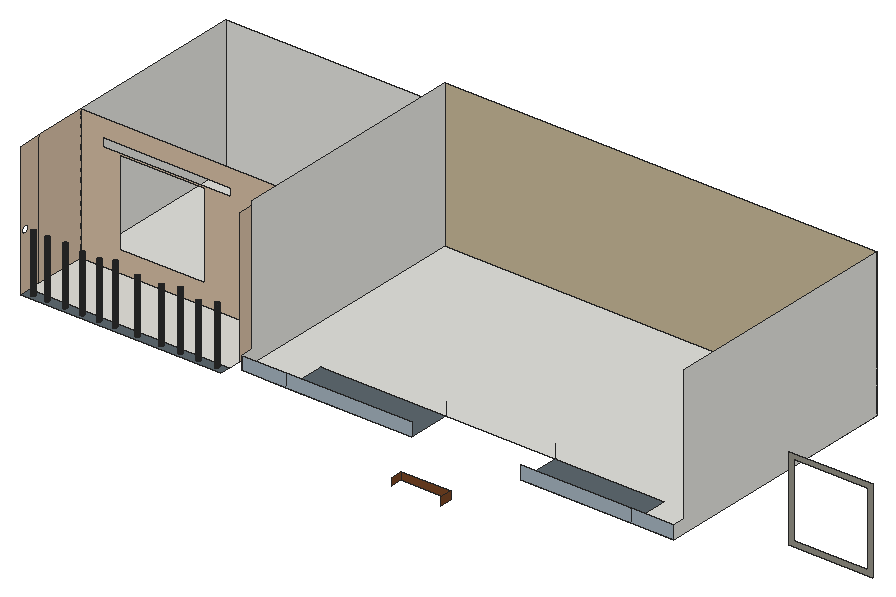
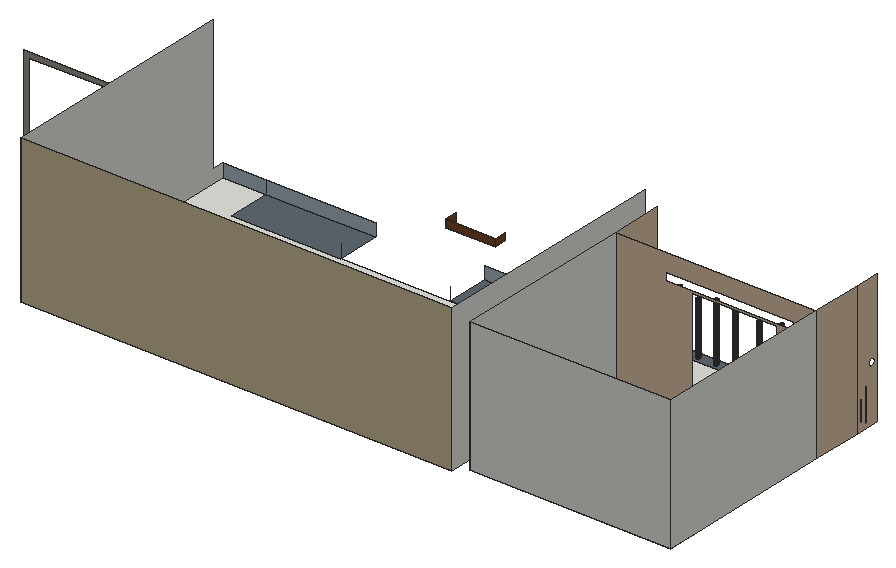
# SketchUp Ruby script. Lengths in inches.
U = 1.inch
M = Sketchup.active_model
def pt(a) = Geom::Point3d.new(a.map { |v| v * U })
def face(e, loops, mat)
  f = e.add_face(loops[0].map { |a| pt(a) })
  loops[1..].each { |l| e.add_face(l.map { |a| pt(a) }).erase! }
  f.material = f.back_material = mat if mat
  f
end
# faces: each face lists its corners as indices into pts; further lists are holes
def faces(e, pts, list, mat = nil) = list.each { |f| face(e, (f[0].is_a?(Array) ? f : [f]).map { |l| l.map { |i| pts[i] } }, mat) }
# xy, xz, yz: faces in a plane at the given z, y or x. An outline is a flat list of corners, or four numbers for a rectangle; further outlines are holes
def ring(l) = l.size == 4 ? [[l[0], l[1]], [l[2], l[1]], [l[2], l[3]], [l[0], l[3]]] : l.each_slice(2).to_a
def flat(e, list, mat, &to3) = list.each { |f| face(e, (f[0].is_a?(Array) ? f : [f]).map { |l| ring(l).map { |u, v| to3.(u, v) } }, mat) }
def xy(e, z, list, mat = nil) = flat(e, list, mat) { |x, y| [x, y, z] }
def xz(e, y, list, mat = nil) = flat(e, list, mat) { |x, z| [x, y, z] }
def yz(e, x, list, mat = nil) = flat(e, list, mat) { |y, z| [x, y, z] }
def lines(e, pts, list) = list.each { |a, b| e.add_line(pt(pts[a]), pt(pts[b])) }
# prism: a flat outline (further loops are holes) pulled along v
def prism(e, loops, v, mat = nil)
  f = face(e, loops, mat); d = Geom::Vector3d.new(v.map { |x| x * U })
  f.pushpull(f.normal.samedirection?(d) ? d.length : -d.length)
end
def box(e, o, s, mat = nil) = prism(e, [[o, [o[0] + s[0], o[1], o[2]], [o[0] + s[0], o[1] + s[1], o[2]], [o[0], o[1] + s[1], o[2]]]], [0, 0, s[2]], mat)
def at(x, y, z, deg = 0) = Geom::Transformation.translation(pt([x, y, z])) * Geom::Transformation.rotation(ORIGIN, Z_AXIS, deg.degrees)
def axes(o, x, y, z) = Geom::Transformation.new([*x, 0, *y, 0, *z, 0, *pt(o).to_a, 1])
def part(name) = M.definitions.add(name)
# library, detail: a bought-in or finely detailed component or shape, given as its bounding box
def library(name, o, s) = part(name).tap { |d| box(d.entities, o, s) }
def detail(e, o, s) = box(e.add_group.entities, o, s)
def put(e, d, t, mat = nil) = e.add_instance(d, t).tap { |i| i.material = mat if mat }
def group(e, t, mat = nil) = e.add_group.tap { |g| g.transformation = t; g.material = mat if mat }.entities
root = M.entities
M.materials.add("[Formica Graystone]").color = [149, 146, 135]
M.materials.add("[Formica Laminate Dark]").color = [50, 53, 60]
M.materials.add("[Formica Laminate Light]").color = [213, 189, 164]
M.materials.add("[Formica Speckled Grey]").color = [94, 105, 111]
M.materials.add("[Marble Carrara Gold Floor Tile]").color = [225, 223, 217]
M.materials.add("[Quartz Light Brown]").color = [199, 184, 152]
M.materials.add("[Terrazzo Light Blue]1").color = [165, 180, 191]
M.materials.add("[Wood Veneer 01]2").color = [120, 70, 37]
xy(root,513,[[16.13,126.7,15.66,126.76,15.22,126.95,14.85,127.23,14.56,127.61,14.375,128.05,14.31,128.51,14.375,128.98,14.56,129.42,14.85,129.8,15.22,130.08,15.66,130.27,16.13,130.33,16.6,130.27,17.03,130.08,17.41,129.8,17.7,129.42,17.88,128.98,17.94,128.51,17.88,128.05,17.7,127.61,17.41,127.23,17.03,126.95,16.6,126.76],[29.13,126.7,28.66,126.76,28.22,126.95,27.85,127.23,27.56,127.61,27.375,128.05,27.31,128.51,27.375,128.98,27.56,129.42,27.85,129.8,28.22,130.08,28.66,130.27,29.13,130.33,29.6,130.27,30.03,130.08,30.41,129.8,30.7,129.42,30.88,128.98,30.94,128.51,30.88,128.05,30.7,127.61,30.41,127.23,30.03,126.95,29.6,126.76],[44.81,126.7,44.35,126.76,43.91,126.95,43.53,127.23,43.25,127.61,43.0625,128.05,43,128.51,43.0625,128.98,43.25,129.42,43.53,129.8,43.91,130.08,44.35,130.27,44.81,130.33,45.28,130.27,45.72,130.08,46.1,129.8,46.38,129.42,46.57,128.98,46.63,128.51,46.57,128.05,46.38,127.61,46.1,127.23,45.72,126.95,45.28,126.76],[60.69,126.7,60.22,126.76,59.78,126.95,59.41,127.23,59.12,127.61,58.9375,128.05,58.88,128.51,58.9375,128.98,59.12,129.42,59.41,129.8,59.78,130.08,60.22,130.27,60.69,130.33,61.16,130.27,61.6,130.08,61.97,129.8,62.26,129.42,62.44,128.98,62.5,128.51,62.44,128.05,62.26,127.61,61.97,127.23,61.6,126.95,61.16,126.76],[75.69,126.7,75.22,126.76,74.78,126.95,74.41,127.23,74.12,127.61,73.9375,128.05,73.88,128.51,73.9375,128.98,74.12,129.42,74.41,129.8,74.78,130.08,75.22,130.27,75.69,130.33,76.16,130.27,76.6,130.08,76.97,129.8,77.26,129.42,77.44,128.98,77.5,128.51,77.44,128.05,77.26,127.61,76.97,127.23,76.6,126.95,76.16,126.76],
  [89.81,126.7,89.35,126.76,88.91,126.95,88.53,127.23,88.25,127.61,88.0625,128.05,88,128.51,88.0625,128.98,88.25,129.42,88.53,129.8,88.91,130.08,89.35,130.27,89.81,130.33,90.28,130.27,90.72,130.08,91.1,129.8,91.38,129.42,91.57,128.98,91.63,128.51,91.57,128.05,91.38,127.61,91.1,127.23,90.72,126.95,90.28,126.76],[110.19,126.7,109.72,126.76,109.28,126.95,108.91,127.23,108.62,127.61,108.4375,128.05,108.38,128.51,108.4375,128.98,108.62,129.42,108.91,129.8,109.28,130.08,109.72,130.27,110.19,130.33,110.66,130.27,111.1,130.08,111.47,129.8,111.76,129.42,111.94,128.98,112,128.51,111.94,128.05,111.76,127.61,111.47,127.23,111.1,126.95,110.66,126.76],[131.69,126.7,131.22,126.76,130.78,126.95,130.41,127.23,130.12,127.61,129.9375,128.05,129.88,128.51,129.9375,128.98,130.12,129.42,130.41,129.8,130.78,130.08,131.22,130.27,131.69,130.33,132.16,130.27,132.6,130.08,132.97,129.8,133.26,129.42,133.44,128.98,133.5,128.51,133.44,128.05,133.26,127.61,132.97,127.23,132.6,126.95,132.16,126.76],[149.06,126.7,148.6,126.76,148.16,126.95,147.78,127.23,147.5,127.61,147.3125,128.05,147.25,128.51,147.3125,128.98,147.5,129.42,147.78,129.8,148.16,130.08,148.6,130.27,149.06,130.33,149.53,130.27,149.97,130.08,150.35,129.8,150.63,129.42,150.82,128.98,150.88,128.51,150.82,128.05,150.63,127.61,150.35,127.23,149.97,126.95,149.53,126.76],[165.13,126.7,164.66,126.76,164.22,126.95,163.85,127.23,163.56,127.61,163.375,128.05,163.31,128.51,163.375,128.98,163.56,129.42,163.85,129.8,164.22,130.08,164.66,130.27,165.13,130.33,165.6,130.27,166.03,130.08,166.41,129.8,166.7,129.42,166.88,128.98,166.94,128.51,166.88,128.05,166.7,127.61,166.41,127.23,166.03,126.95,165.6,126.76],
  [181.81,126.7,181.35,126.76,180.91,126.95,180.53,127.23,180.25,127.61,180.0625,128.05,180,128.51,180.0625,128.98,180.25,129.42,180.53,129.8,180.91,130.08,181.35,130.27,181.81,130.33,182.28,130.27,182.72,130.08,183.1,129.8,183.38,129.42,183.57,128.98,183.63,128.51,183.57,128.05,183.38,127.61,183.1,127.23,182.72,126.95,182.28,126.76],[198.57,135.71,198.57,364.125,588.3,364.125,588.3,135.71,549.2,135.71,549.2,174.4375,238.58,174.4375,238.58,135.71],[9,191.15,189.57,355.125]])
xy(root,513,[[[9,122.79,189.57,133.5],[181.81,126.7,181.35,126.76,180.91,126.95,180.53,127.23,180.25,127.61,180.0625,128.05,180,128.51,180.0625,128.98,180.25,129.42,180.53,129.8,180.91,130.08,181.35,130.27,181.81,130.33,182.28,130.27,182.72,130.08,183.1,129.8,183.38,129.42,183.57,128.98,183.63,128.51,183.57,128.05,183.38,127.61,183.1,127.23,182.72,126.95,182.28,126.76],[29.13,126.7,28.66,126.76,28.22,126.95,27.85,127.23,27.56,127.61,27.375,128.05,27.31,128.51,27.375,128.98,27.56,129.42,27.85,129.8,28.22,130.08,28.66,130.27,29.13,130.33,29.6,130.27,30.03,130.08,30.41,129.8,30.7,129.42,30.88,128.98,30.94,128.51,30.88,128.05,30.7,127.61,30.41,127.23,30.03,126.95,29.6,126.76],[165.13,126.7,164.66,126.76,164.22,126.95,163.85,127.23,163.56,127.61,163.375,128.05,163.31,128.51,163.375,128.98,163.56,129.42,163.85,129.8,164.22,130.08,164.66,130.27,165.13,130.33,165.6,130.27,166.03,130.08,166.41,129.8,166.7,129.42,166.88,128.98,166.94,128.51,166.88,128.05,166.7,127.61,166.41,127.23,166.03,126.95,165.6,126.76],[44.81,126.7,44.35,126.76,43.91,126.95,43.53,127.23,43.25,127.61,43.0625,128.05,43,128.51,43.0625,128.98,43.25,129.42,43.53,129.8,43.91,130.08,44.35,130.27,44.81,130.33,45.28,130.27,45.72,130.08,46.1,129.8,46.38,129.42,46.57,128.98,46.63,128.51,46.57,128.05,46.38,127.61,46.1,127.23,45.72,126.95,45.28,126.76],[149.06,126.7,148.6,126.76,148.16,126.95,147.78,127.23,147.5,127.61,147.3125,128.05,147.25,128.51,147.3125,128.98,147.5,129.42,147.78,129.8,148.16,130.08,148.6,130.27,149.06,130.33,149.53,130.27,149.97,130.08,150.35,129.8,150.63,129.42,150.82,128.98,150.88,128.51,150.82,128.05,150.63,127.61,150.35,127.23,149.97,126.95,149.53,126.76],[60.69,126.7,60.22,126.76,59.78,126.95,59.41,127.23,59.12,127.61,58.9375,128.05,58.88,128.51,58.9375,128.98,59.12,129.42,59.41,129.8,59.78,130.08,60.22,130.27,60.69,130.33,61.16,130.27,61.6,130.08,61.97,129.8,62.26,129.42,62.44,128.98,62.5,128.51,62.44,128.05,62.26,127.61,61.97,127.23,61.6,126.95,61.16,126.76],[131.69,126.7,131.22,126.76,130.78,126.95,130.41,127.23,130.12,127.61,129.9375,128.05,129.88,128.51,129.9375,128.98,130.12,129.42,130.41,129.8,130.78,130.08,131.22,130.27,131.69,130.33,132.16,130.27,132.6,130.08,132.97,129.8,133.26,129.42,133.44,128.98,133.5,128.51,133.44,128.05,133.26,127.61,132.97,127.23,132.6,126.95,132.16,126.76],[75.69,126.7,75.22,126.76,74.78,126.95,74.41,127.23,74.12,127.61,73.9375,128.05,73.88,128.51,73.9375,128.98,74.12,129.42,74.41,129.8,74.78,130.08,75.22,130.27,75.69,130.33,76.16,130.27,76.6,130.08,76.97,129.8,77.26,129.42,77.44,128.98,77.5,128.51,77.44,128.05,77.26,127.61,76.97,127.23,76.6,126.95,76.16,126.76],[110.19,126.7,109.72,126.76,109.28,126.95,108.91,127.23,108.62,127.61,108.4375,128.05,108.38,128.51,108.4375,128.98,108.62,129.42,108.91,129.8,109.28,130.08,109.72,130.27,110.19,130.33,110.66,130.27,111.1,130.08,111.47,129.8,111.76,129.42,111.94,128.98,112,128.51,111.94,128.05,111.76,127.61,111.47,127.23,111.1,126.95,110.66,126.76],[89.81,126.7,89.35,126.76,88.91,126.95,88.53,127.23,88.25,127.61,88.0625,128.05,88,128.51,88.0625,128.98,88.25,129.42,88.53,129.8,88.91,130.08,89.35,130.27,89.81,130.33,90.28,130.27,90.72,130.08,91.1,129.8,91.38,129.42,91.57,128.98,91.63,128.51,91.57,128.05,91.38,127.61,91.1,127.23,90.72,126.95,90.28,126.76],[16.13,126.7,15.66,126.76,15.22,126.95,14.85,127.23,14.56,127.61,14.375,128.05,14.31,128.51,14.375,128.98,14.56,129.42,14.85,129.8,15.22,130.08,15.66,130.27,16.13,130.33,16.6,130.27,17.03,130.08,17.41,129.8,17.7,129.42,17.88,128.98,17.94,128.51,17.88,128.05,17.7,127.61,17.41,127.23,17.03,126.95,16.6,126.76]],[238.58,135.71,351.88,174.4375],[450.54,135.71,549.2,174.4375]],"[Formica Speckled Grey]")
xy(root,513,[[9,133.5,189.57,191.15]],"[Marble Carrara Gold Floor Tile]")
xz(root,88.2,[[380.3,508.89,424.94,515.72]],"[Wood Veneer 01]2")
xz(root,135.71,[[198.57,513,238.58,525],[238.58,513,351.88,525],[450.54,513,549.2,525],[549.2,513,588.3,525]],"[Terrazzo Light Blue]1")
xz(root,182.57,[[[654.83,511.625,730.21,587],[659.44,516.23,725.6,582.39]]],"[Formica Graystone]")
xz(root,191.15,[[[9,513,189.57,633],[43.9375,531.79,120.375,608.22],[28.72,609.74,143.97,617.3]]],"[Formica Laminate Light]")
xz(root,355.125,[[9,513,189.57,633]])
xz(root,364.125,[[198.57,513,588.3,645]],"[Quartz Light Brown]")
yz(root,9,[[191.15,513,355.125,633]])
yz(root,9,[[[122.79,513,144.21,633],[128.15,560.5625,127.31,560.67,126.52,561,125.85,561.51,125.33,562.1875,125.01,562.97,124.9,563.8125,125.01,564.65,125.33,565.4375,125.85,566.11,126.52,566.625,127.31,566.95,128.15,567.0625,128.99,566.95,129.77,566.625,130.45,566.11,130.96,565.4375,131.29,564.65,131.4,563.8125,131.29,562.97,130.96,562.1875,130.45,561.51,129.77,561,128.99,560.67]],[144.21,513,191.15,633]],"[Formica Laminate Light]")
yz(root,189.57,[[191.15,513,355.125,633]])
yz(root,189.57,[[144.21,513,191.15,633]],"[Formica Laminate Light]")
yz(root,198.57,[[135.71,513,135.71,525,147.05,525,147.05,645,364.125,645,364.125,513]])
yz(root,380.3,[[77.26,508.89,88.2,515.72]],"[Wood Veneer 01]2")
yz(root,424.94,[[77.26,508.89,88.2,515.72]],"[Wood Veneer 01]2")
yz(root,588.3,[[135.71,513,135.71,525,147.05,525,147.05,645,364.125,645,364.125,513]])
p = [[15.66,126.76,513],[16.13,126.7,513],[16.13,126.7,564.65],[15.66,126.76,564.65],[16.6,126.76,513],[16.6,126.76,564.65],
  [28.66,126.76,513],[29.13,126.7,513],[29.13,126.7,564.0625],[28.66,126.76,564.0625],[29.6,126.76,513],[29.6,126.76,564.0625],
  [44.35,126.76,513],[44.81,126.7,513],[44.81,126.7,564.5625],[44.35,126.76,564.5625],[45.28,126.76,513],[45.28,126.76,564.5625],
  [60.22,126.76,513],[60.69,126.7,513],[60.69,126.7,562.9375],[60.22,126.76,562.9375],[61.16,126.76,513],[61.16,126.76,562.9375],
  [75.22,126.76,513],[75.69,126.7,513],[75.69,126.7,562.6875],[75.22,126.76,562.6875],[76.16,126.76,513],[76.16,126.76,562.6875],
  [89.35,126.76,513],[89.81,126.7,513],[89.81,126.7,566.11],[89.35,126.76,566.11],[90.28,126.76,513],[90.28,126.76,566.11],
  [109.72,126.76,513],[110.19,126.7,513],[110.19,126.7,561.5],[109.72,126.76,561.5],[110.66,126.76,513],[110.66,126.76,561.5],
  [131.22,126.76,513],[131.69,126.7,513],[131.69,126.7,561.8125],[131.22,126.76,561.8125],[132.16,126.76,513],[132.16,126.76,561.8125],
  [148.6,126.76,513],[149.06,126.7,513],[149.06,126.7,565.4375],[148.6,126.76,565.4375],[149.53,126.76,513],[149.53,126.76,565.4375],
  [164.66,126.76,513],[165.13,126.7,513],[165.13,126.7,560.5625],[164.66,126.76,560.5625],[165.6,126.76,513],[165.6,126.76,560.5625],
  [181.35,126.76,513],[181.81,126.7,513],[181.81,126.7,564.65],[181.35,126.76,564.65],[182.28,126.76,513],[182.28,126.76,564.65],
  [15.22,126.95,513],[15.22,126.95,564.65],[17.03,126.95,513],[17.03,126.95,564.65],[28.22,126.95,513],[28.22,126.95,564.0625],
  [30.03,126.95,513],[30.03,126.95,564.0625],[43.91,126.95,513],[43.91,126.95,564.5625],[45.72,126.95,513],[45.72,126.95,564.5625],
  [59.78,126.95,513],[59.78,126.95,562.9375],[61.6,126.95,513],[61.6,126.95,562.9375],[74.78,126.95,513],[74.78,126.95,562.6875],
  [76.6,126.95,513],[76.6,126.95,562.6875],[88.91,126.95,513],[88.91,126.95,566.11],[90.72,126.95,513],[90.72,126.95,566.11],
  [109.28,126.95,513],[109.28,126.95,561.5],[111.1,126.95,513],[111.1,126.95,561.5],[130.78,126.95,513],[130.78,126.95,561.8125],
  [132.6,126.95,513],[132.6,126.95,561.8125],[148.16,126.95,513],[148.16,126.95,565.4375],[149.97,126.95,513],[149.97,126.95,565.4375],
  [164.22,126.95,513],[164.22,126.95,560.5625],[166.03,126.95,513],[166.03,126.95,560.5625],[180.91,126.95,513],[180.91,126.95,564.65],
  [182.72,126.95,513],[182.72,126.95,564.65],[14.85,127.23,513],[14.85,127.23,564.65],[17.41,127.23,513],[17.41,127.23,564.65],
  [27.85,127.23,513],[27.85,127.23,564.0625],[30.41,127.23,513],[30.41,127.23,564.0625],[43.53,127.23,513],[43.53,127.23,564.5625],
  [46.1,127.23,513],[46.1,127.23,564.5625],[59.41,127.23,513],[59.41,127.23,562.9375],[61.97,127.23,513],[61.97,127.23,562.9375],
  [74.41,127.23,513],[74.41,127.23,562.6875],[76.97,127.23,513],[76.97,127.23,562.6875],[88.53,127.23,513],[88.53,127.23,566.11],
  [91.1,127.23,513],[91.1,127.23,566.11],[108.91,127.23,513],[108.91,127.23,561.5],[111.47,127.23,513],[111.47,127.23,561.5],
  [130.41,127.23,513],[130.41,127.23,561.8125],[132.97,127.23,513],[132.97,127.23,561.8125],[147.78,127.23,513],[147.78,127.23,565.4375],
  [150.35,127.23,513],[150.35,127.23,565.4375],[163.85,127.23,513],[163.85,127.23,560.5625],[166.41,127.23,513],[166.41,127.23,560.5625],
  [180.53,127.23,513],[180.53,127.23,564.65],[183.1,127.23,513],[183.1,127.23,564.65],[14.56,127.61,513],[14.56,127.61,564.65],
  [17.7,127.61,513],[17.7,127.61,564.65],[27.56,127.61,513],[27.56,127.61,564.0625],[30.7,127.61,513],[30.7,127.61,564.0625],
  [43.25,127.61,513],[43.25,127.61,564.5625],[46.38,127.61,513],[46.38,127.61,564.5625],[59.12,127.61,513],[59.12,127.61,562.9375],
  [62.26,127.61,513],[62.26,127.61,562.9375],[74.12,127.61,513],[74.12,127.61,562.6875],[77.26,127.61,513],[77.26,127.61,562.6875],
  [88.25,127.61,513],[88.25,127.61,566.11],[91.38,127.61,513],[91.38,127.61,566.11],[108.62,127.61,513],[108.62,127.61,561.5],
  [111.76,127.61,513],[111.76,127.61,561.5],[130.12,127.61,513],[130.12,127.61,561.8125],[133.26,127.61,513],[133.26,127.61,561.8125],
  [147.5,127.61,513],[147.5,127.61,565.4375],[150.63,127.61,513],[150.63,127.61,565.4375],[163.56,127.61,513],[163.56,127.61,560.5625],
  [166.7,127.61,513],[166.7,127.61,560.5625],[180.25,127.61,513],[180.25,127.61,564.65],[183.38,127.61,513],[183.38,127.61,564.65],
  [14.375,128.05,513],[14.375,128.05,564.65],[17.88,128.05,513],[17.88,128.05,564.65],[27.375,128.05,513],[27.375,128.05,564.0625],
  [30.88,128.05,513],[30.88,128.05,564.0625],[43.0625,128.05,513],[43.0625,128.05,564.5625],[46.57,128.05,513],[46.57,128.05,564.5625],
  [58.9375,128.05,513],[58.9375,128.05,562.9375],[62.44,128.05,513],[62.44,128.05,562.9375],[73.9375,128.05,513],[73.9375,128.05,562.6875],
  [77.44,128.05,513],[77.44,128.05,562.6875],[88.0625,128.05,513],[88.0625,128.05,566.11],[91.57,128.05,513],[91.57,128.05,566.11],
  [108.4375,128.05,513],[108.4375,128.05,561.5],[111.94,128.05,513],[111.94,128.05,561.5],[129.9375,128.05,513],[129.9375,128.05,561.8125],
  [133.44,128.05,513],[133.44,128.05,561.8125],[147.3125,128.05,513],[147.3125,128.05,565.4375],[150.82,128.05,513],[150.82,128.05,565.4375],
  [163.375,128.05,513],[163.375,128.05,560.5625],[166.88,128.05,513],[166.88,128.05,560.5625],[180.0625,128.05,513],[180.0625,128.05,564.65],
  [183.57,128.05,513],[183.57,128.05,564.65],[14.31,128.51,513],[14.31,128.51,564.65],[17.94,128.51,513],[17.94,128.51,564.65],
  [27.31,128.51,513],[27.31,128.51,564.0625],[30.94,128.51,513],[30.94,128.51,564.0625],[43,128.51,513],[43,128.51,564.5625],
  [46.63,128.51,513],[46.63,128.51,564.5625],[58.88,128.51,513],[58.88,128.51,562.9375],[62.5,128.51,513],[62.5,128.51,562.9375],
  [73.88,128.51,513],[73.88,128.51,562.6875],[77.5,128.51,513],[77.5,128.51,562.6875],[88,128.51,513],[88,128.51,566.11],
  [91.63,128.51,513],[91.63,128.51,566.11],[108.38,128.51,513],[108.38,128.51,561.5],[112,128.51,513],[112,128.51,561.5],
  [129.88,128.51,513],[129.88,128.51,561.8125],[133.5,128.51,513],[133.5,128.51,561.8125],[147.25,128.51,513],[147.25,128.51,565.4375],
  [150.88,128.51,513],[150.88,128.51,565.4375],[163.31,128.51,513],[163.36,128.15,560.5625],[163.31,128.51,560.5625],[166.94,128.51,513],
  [166.94,128.51,560.5625],[166.89,128.15,560.5625],[180,128.51,513],[180,128.51,564.65],[183.63,128.51,513],[183.63,128.51,564.65],
  [14.375,128.98,513],[14.375,128.98,564.65],[17.88,128.98,513],[17.88,128.98,564.65],[27.375,128.98,513],[27.375,128.98,564.0625],
  [30.88,128.98,513],[30.88,128.98,564.0625],[43.0625,128.98,513],[43.0625,128.98,564.5625],[46.57,128.98,513],[46.57,128.98,564.5625],
  [58.9375,128.98,513],[58.9375,128.98,562.9375],[62.44,128.98,513],[62.44,128.98,562.9375],[73.9375,128.98,513],[73.9375,128.98,562.6875],
  [77.44,128.98,513],[77.44,128.98,562.6875],[88.0625,128.98,513],[88.0625,128.98,566.11],[91.57,128.98,513],[91.57,128.98,566.11],
  [108.4375,128.98,513],[108.4375,128.98,561.5],[111.94,128.98,513],[111.94,128.98,561.5],[129.9375,128.98,513],[129.9375,128.98,561.8125],
  [133.44,128.98,513],[133.44,128.98,561.8125],[147.3125,128.98,513],[147.3125,128.98,565.4375],[150.82,128.98,513],[150.82,128.98,565.4375],
  [163.375,128.98,513],[163.375,128.98,560.5625],[166.88,128.98,513],[166.88,128.98,560.5625],[180.0625,128.98,513],[180.0625,128.98,564.65],
  [183.57,128.98,513],[183.57,128.98,564.65],[14.56,129.42,513],[14.56,129.42,564.65],[17.7,129.42,513],[17.7,129.42,564.65],
  [27.56,129.42,513],[27.56,129.42,564.0625],[30.7,129.42,513],[30.7,129.42,564.0625],[43.25,129.42,513],[43.25,129.42,564.5625],
  [46.38,129.42,513],[46.38,129.42,564.5625],[59.12,129.42,513],[59.12,129.42,562.9375],[62.26,129.42,513],[62.26,129.42,562.9375],
  [74.12,129.42,513],[74.12,129.42,562.6875],[77.26,129.42,513],[77.26,129.42,562.6875],[88.25,129.42,513],[88.25,129.42,566.11],
  [91.38,129.42,513],[91.38,129.42,566.11],[108.62,129.42,513],[108.62,129.42,561.5],[111.76,129.42,513],[111.76,129.42,561.5],
  [130.12,129.42,513],[130.12,129.42,561.8125],[133.26,129.42,513],[133.26,129.42,561.8125],[147.5,129.42,513],[147.5,129.42,565.4375],
  [150.63,129.42,513],[150.63,129.42,565.4375],[163.56,129.42,513],[163.56,129.42,560.5625],[166.7,129.42,513],[166.7,129.42,560.5625],
  [180.25,129.42,513],[180.25,129.42,564.65],[183.38,129.42,513],[183.38,129.42,564.65],[14.85,129.8,513],[14.85,129.8,564.65],
  [17.41,129.8,513],[17.41,129.8,564.65],[27.85,129.8,513],[27.85,129.8,564.0625],[30.41,129.8,513],[30.41,129.8,564.0625],
  [43.53,129.8,513],[43.53,129.8,564.5625],[46.1,129.8,513],[46.1,129.8,564.5625],[59.41,129.8,513],[59.41,129.8,562.9375],
  [61.97,129.8,513],[61.97,129.8,562.9375],[74.41,129.8,513],[74.41,129.8,562.6875],[76.97,129.8,513],[76.97,129.8,562.6875],
  [88.53,129.8,513],[88.53,129.8,566.11],[91.1,129.8,513],[91.1,129.8,566.11],[108.91,129.8,513],[108.91,129.8,561.5],
  [111.47,129.8,513],[111.47,129.8,561.5],[130.41,129.8,513],[130.41,129.8,561.8125],[132.97,129.8,513],[132.97,129.8,561.8125],
  [147.78,129.8,513],[147.78,129.8,565.4375],[150.35,129.8,513],[150.35,129.8,565.4375],[163.85,129.8,513],[163.85,129.8,560.5625],
  [166.41,129.8,513],[166.41,129.8,560.5625],[180.53,129.8,513],[180.53,129.8,564.65],[183.1,129.8,513],[183.1,129.8,564.65],
  [15.22,130.08,513],[15.22,130.08,564.65],[17.03,130.08,513],[17.03,130.08,564.65],[28.22,130.08,513],[28.22,130.08,564.0625],
  [30.03,130.08,513],[30.03,130.08,564.0625],[43.91,130.08,513],[43.91,130.08,564.5625],[45.72,130.08,513],[45.72,130.08,564.5625],
  [59.78,130.08,513],[59.78,130.08,562.9375],[61.6,130.08,513],[61.6,130.08,562.9375],[74.78,130.08,513],[74.78,130.08,562.6875],
  [76.6,130.08,513],[76.6,130.08,562.6875],[88.91,130.08,513],[88.91,130.08,566.11],[90.72,130.08,513],[90.72,130.08,566.11],
  [109.28,130.08,513],[109.28,130.08,561.5],[111.1,130.08,513],[111.1,130.08,561.5],[130.78,130.08,513],[130.78,130.08,561.8125],
  [132.6,130.08,513],[132.6,130.08,561.8125],[148.16,130.08,513],[148.16,130.08,565.4375],[149.97,130.08,513],[149.97,130.08,565.4375],
  [164.22,130.08,513],[164.22,130.08,560.5625],[166.03,130.08,513],[166.03,130.08,560.5625],[180.91,130.08,513],[180.91,130.08,564.65],
  [182.72,130.08,513],[182.72,130.08,564.65],[15.66,130.27,513],[15.66,130.27,564.65],[16.6,130.27,513],[16.6,130.27,564.65],
  [28.66,130.27,513],[28.66,130.27,564.0625],[29.6,130.27,513],[29.6,130.27,564.0625],[44.35,130.27,513],[44.35,130.27,564.5625],
  [45.28,130.27,513],[45.28,130.27,564.5625],[60.22,130.27,513],[60.22,130.27,562.9375],[61.16,130.27,513],[61.16,130.27,562.9375],
  [75.22,130.27,513],[75.22,130.27,562.6875],[76.16,130.27,513],[76.16,130.27,562.6875],[89.35,130.27,513],[89.35,130.27,566.11],
  [90.28,130.27,513],[90.28,130.27,566.11],[109.72,130.27,513],[109.72,130.27,561.5],[110.66,130.27,513],[110.66,130.27,561.5],
  [131.22,130.27,513],[131.22,130.27,561.8125],[132.16,130.27,513],[132.16,130.27,561.8125],[148.6,130.27,513],[148.6,130.27,565.4375],
  [149.53,130.27,513],[149.53,130.27,565.4375],[164.66,130.27,513],[164.66,130.27,560.5625],[165.6,130.27,513],[165.6,130.27,560.5625],
  [181.35,130.27,513],[181.35,130.27,564.65],[182.28,130.27,513],[182.28,130.27,564.65],[16.13,130.33,513],[16.13,130.33,564.65],
  [29.13,130.33,513],[29.13,130.33,564.0625],[44.81,130.33,513],[44.81,130.33,564.5625],[60.69,130.33,513],[60.69,130.33,562.9375],
  [75.69,130.33,513],[75.69,130.33,562.6875],[89.81,130.33,513],[89.81,130.33,566.11],[110.19,130.33,513],[110.19,130.33,561.5],
  [131.69,130.33,513],[131.69,130.33,561.8125],[149.06,130.33,513],[149.06,130.33,565.4375],[165.13,130.33,513],[165.13,130.33,560.5625],
  [181.81,130.33,513],[181.81,130.33,564.65],[351.88,174.4375,513],[351.88,174.4375,525],[450.54,174.4375,513],[450.54,174.4375,525]]
faces(root,p,[[0,1,2,3],[1,4,5,2],[6,7,8,9],[7,10,11,8],[12,13,14,15],[13,16,17,14],[18,19,20,21],[19,22,23,20],
  [24,25,26,27],[25,28,29,26],[30,31,32,33],[31,34,35,32],[36,37,38,39],[37,40,41,38],[42,43,44,45],[43,46,47,44],
  [48,49,50,51],[49,52,53,50],[54,55,56,57],[55,58,59,56],[60,61,62,63],[61,64,65,62],[66,0,3,67],[4,68,69,5],
  [70,6,9,71],[10,72,73,11],[74,12,15,75],[16,76,77,17],[78,18,21,79],[22,80,81,23],[82,24,27,83],[28,84,85,29],
  [86,30,33,87],[34,88,89,35],[90,36,39,91],[40,92,93,41],[94,42,45,95],[46,96,97,47],[98,48,51,99],[52,100,101,53],
  [102,54,57,103],[58,104,105,59],[106,60,63,107],[64,108,109,65],[110,66,67,111],[68,112,113,69],[114,70,71,115],[72,116,117,73],
  [118,74,75,119],[76,120,121,77],[122,78,79,123],[80,124,125,81],[126,82,83,127],[84,128,129,85],[130,86,87,131],[88,132,133,89],
  [134,90,91,135],[92,136,137,93],[138,94,95,139],[96,140,141,97],[142,98,99,143],[100,144,145,101],[146,102,103,147],[104,148,149,105],
  [150,106,107,151],[108,152,153,109],[154,110,111,155],[112,156,157,113],[158,114,115,159],[116,160,161,117],[162,118,119,163],[120,164,165,121],
  [166,122,123,167],[124,168,169,125],[170,126,127,171],[128,172,173,129],[174,130,131,175],[132,176,177,133],[178,134,135,179],[136,180,181,137],
  [182,138,139,183],[140,184,185,141],[186,142,143,187],[144,188,189,145],[190,146,147,191],[148,192,193,149],[194,150,151,195],[152,196,197,153],
  [198,154,155,199],[156,200,201,157],[202,158,159,203],[160,204,205,161],[206,162,163,207],[164,208,209,165],[210,166,167,211],[168,212,213,169],
  [214,170,171,215],[172,216,217,173],[218,174,175,219],[176,220,221,177],[222,178,179,223],[180,224,225,181],[226,182,183,227],[184,228,229,185],
  [230,186,187,231],[188,232,233,189],[234,190,191,235],[192,236,237,193],[238,194,195,239],[196,240,241,197],[242,198,199,243],[200,244,245,201],
  [246,202,203,247],[204,248,249,205],[250,206,207,251],[208,252,253,209],[254,210,211,255],[212,256,257,213],[258,214,215,259],[216,260,261,217],
  [262,218,219,263],[220,264,265,221],[266,222,223,267],[224,268,269,225],[270,226,227,271],[228,272,273,229],[274,230,231,275],[232,276,277,233],
  [278,234,235,279,280],[236,281,282,283,237],[284,238,239,285],[240,286,287,241],[288,242,243,289],[244,290,291,245],[292,246,247,293],[248,294,295,249],
  [296,250,251,297],[252,298,299,253],[300,254,255,301],[256,302,303,257],[304,258,259,305],[260,306,307,261],[308,262,263,309],[264,310,311,265],
  [312,266,267,313],[268,314,315,269],[316,270,271,317],[272,318,319,273],[320,274,275,321],[276,322,323,277],[324,278,280,325],[281,326,327,282],
  [328,284,285,329],[286,330,331,287],[332,288,289,333],[290,334,335,291],[336,292,293,337],[294,338,339,295],[340,296,297,341],[298,342,343,299],
  [344,300,301,345],[302,346,347,303],[348,304,305,349],[306,350,351,307],[352,308,309,353],[310,354,355,311],[356,312,313,357],[314,358,359,315],
  [360,316,317,361],[318,362,363,319],[364,320,321,365],[322,366,367,323],[368,324,325,369],[326,370,371,327],[372,328,329,373],[330,374,375,331],
  [376,332,333,377],[334,378,379,335],[380,336,337,381],[338,382,383,339],[384,340,341,385],[342,386,387,343],[388,344,345,389],[346,390,391,347],
  [392,348,349,393],[350,394,395,351],[396,352,353,397],[354,398,399,355],[400,356,357,401],[358,402,403,359],[404,360,361,405],[362,406,407,363],
  [408,364,365,409],[366,410,411,367],[412,368,369,413],[370,414,415,371],[416,372,373,417],[374,418,419,375],[420,376,377,421],[378,422,423,379],
  [424,380,381,425],[382,426,427,383],[428,384,385,429],[386,430,431,387],[432,388,389,433],[390,434,435,391],[436,392,393,437],[394,438,439,395],
  [440,396,397,441],[398,442,443,399],[444,400,401,445],[402,446,447,403],[448,404,405,449],[406,450,451,407],[452,408,409,453],[410,454,455,411],
  [456,412,413,457],[414,458,459,415],[460,416,417,461],[418,462,463,419],[464,420,421,465],[422,466,467,423],[468,424,425,469],[426,470,471,427],
  [472,428,429,473],[430,474,475,431],[476,432,433,477],[434,478,479,435],[480,436,437,481],[438,482,483,439],[484,440,441,485],[442,486,487,443],
  [488,444,445,489],[446,490,491,447],[492,448,449,493],[450,494,495,451],[496,452,453,497],[454,498,499,455],[500,456,457,501],[458,502,503,459],
  [504,460,461,505],[462,506,507,463],[508,464,465,509],[466,508,509,467],[510,468,469,511],[470,510,511,471],[512,472,473,513],[474,512,513,475],
  [514,476,477,515],[478,514,515,479],[516,480,481,517],[482,516,517,483],[518,484,485,519],[486,518,519,487],[520,488,489,521],[490,520,521,491],
  [522,492,493,523],[494,522,523,495],[524,496,497,525],[498,524,525,499],[526,500,501,527],[502,526,527,503],[528,504,505,529],[506,528,529,507]],"[Formica Laminate Dark]")
lines(root,p,[[530,531],[532,533]])
